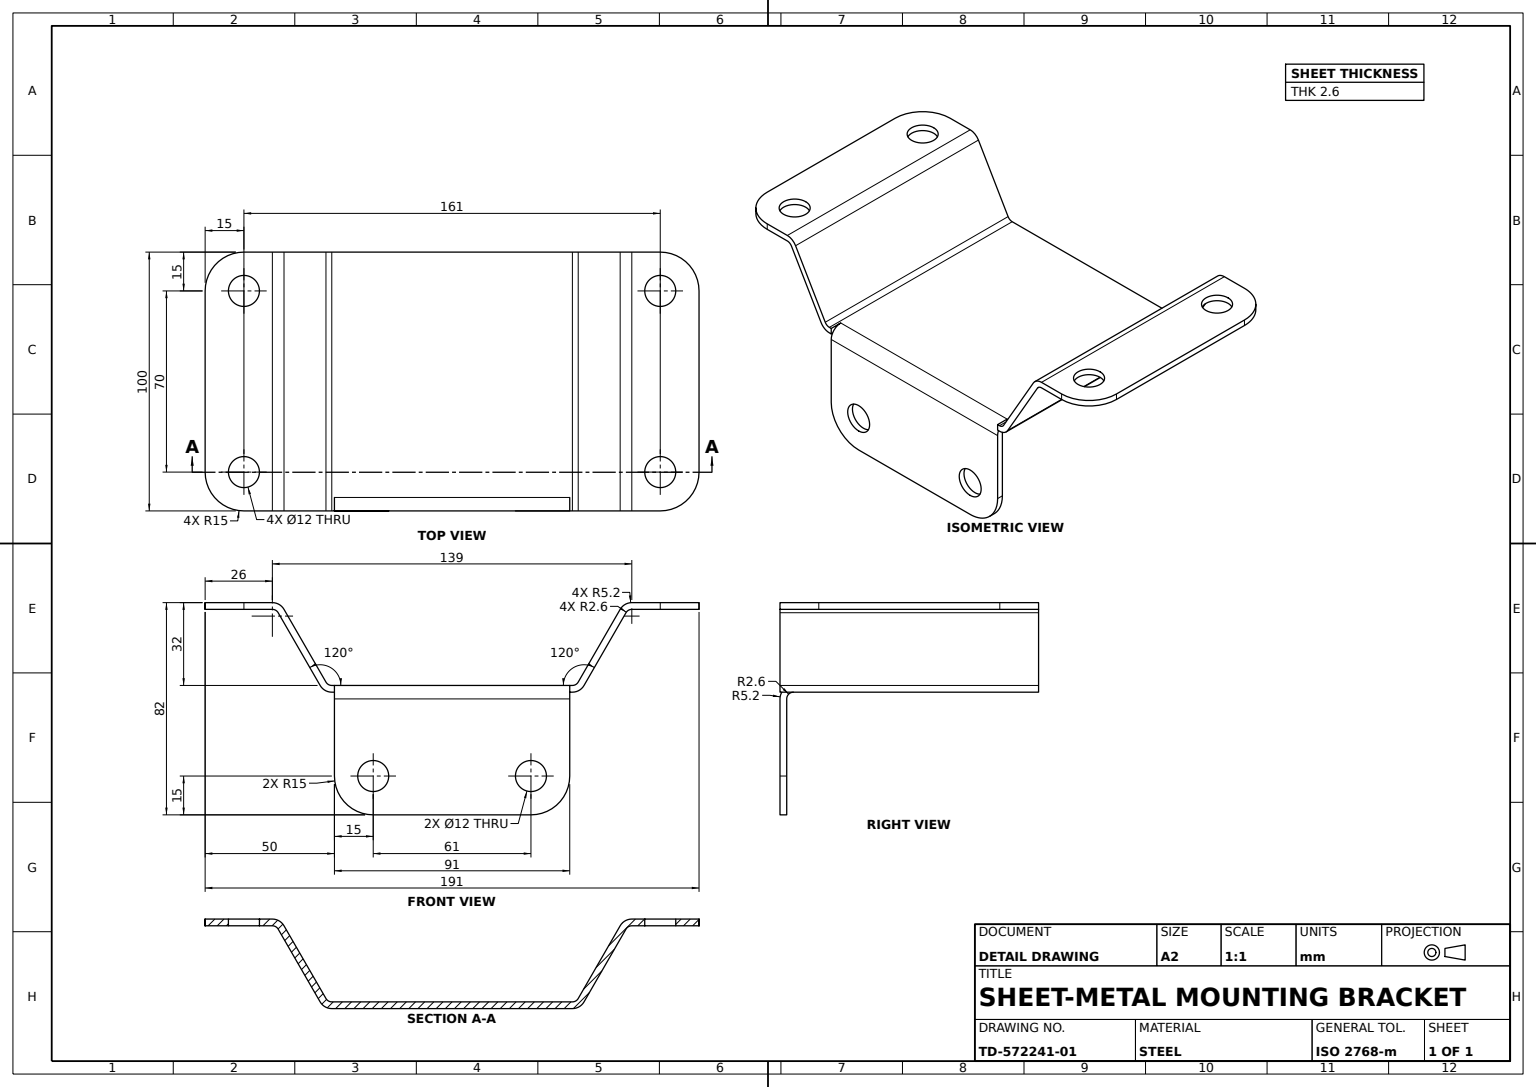
solid
v1 (-51.027013,0,-50)
v2 (-67.250555,28.1,-50)
e1 v1 v2 LINE
v3 (-64.998889,29.4,-50)
e2 v2 v3 LINE
v4 (-48.775347,1.3,-50)
e3 v4 v3 LINE
e4 v4 v1 LINE
face PLANE(AX(P(-46.523681,-2.6,-50),D(0,0,-1),D(-1,0,0))) [e1 e2 -e3 e4]
v5 (-67.250555,28.1,50)
e5 v5 v2 LINE
v6 (-69.502221,29.4,50)
e6 v5 v6 CIRCLE(AX(P(-69.502221,26.8,50),D(0,0,1),D(1,0,0)),2.6)
v7 (-69.502221,29.4,-50)
e7 v6 v7 LINE
e8 v2 v7 CIRCLE(AX(P(-69.502221,26.8,-50),D(0,0,1),D(1,0,0)),2.6)
face CYL(AX(P(-69.502221,26.8,50),D(0,0,-1),D(-1,0,0)),2.6) rev [-e5 e6 e7 -e8]
v8 (45.5,0,50)
v9 (45.5,0,44.8)
e9 v8 v9 LINE
v10 (45.5,-2.6,49.303332)
e10 v9 v10 CIRCLE(AX(P(45.5,-5.2,44.8),D(1,0,0),D(0,0,1)),5.2)
v11 (45.5,-2.6,50)
e11 v10 v11 LINE
e12 v11 v8 LINE
face PLANE(AX(P(45.5,-2.6,44.8),D(-1,0,0),D(0,0,1))) [e9 e10 e11 e12]
v12 (-80.5,29.4,-29)
v13 (-80.5,29.4,-41)
e13 v12 v13 CIRCLE(AX(P(-80.5,29.4,-35),D(0,1,0),D(0,0,1)),6)
v14 (-80.5,32,-29)
e14 v12 v14 LINE
v15 (-80.5,32,-41)
e15 v14 v15 CIRCLE(AX(P(-80.5,32,-35),D(0,1,0),D(0,0,1)),6)
e16 v13 v15 LINE
face CYL(AX(P(-80.5,29.4,-35),D(0,1,0),D(0,0,1)),6) rev [-e13 e14 e15 -e16]
v16 (-64.998889,29.4,50)
v17 (-69.502221,32,50)
e17 v16 v17 CIRCLE(AX(P(-69.502221,26.8,50),D(0,0,1),D(-1,0,0)),5.2)
e18 v16 v3 LINE
v18 (-69.502221,32,-50)
e19 v3 v18 CIRCLE(AX(P(-69.502221,26.8,-50),D(0,0,1),D(-1,0,0)),5.2)
e20 v17 v18 LINE
face CYL(AX(P(-69.502221,26.8,50),D(0,0,-1),D(-1,0,0)),5.2) [-e17 e18 e19 -e20]
v19 (45.5,-5.2,50)
e21 v10 v19 CIRCLE(AX(P(45.5,-5.2,44.8),D(1,0,0),D(0,0,1)),5.2)
v20 (-45.5,0,44.8)
e22 v20 v9 LINE
v21 (-45.5,-2.6,49.303332)
e23 v21 v20 CIRCLE(AX(P(-45.5,-5.2,44.8),D(-1,0,0),D(0,0,1)),5.2)
v22 (-45.5,-5.2,50)
e24 v22 v21 CIRCLE(AX(P(-45.5,-5.2,44.8),D(-1,0,0),D(0,0,1)),5.2)
e25 v22 v19 LINE
face CYL(AX(P(-45.5,-5.2,44.8),D(-1,0,0),D(0,0,1)),5.2) [-e21 -e10 -e22 -e23 -e24 e25]
v23 (51.027013,0,-50)
v24 (48.775347,1.3,-50)
e26 v23 v24 LINE
v25 (46.523681,-2.6,-50)
e27 v23 v25 CIRCLE(AX(P(46.523681,2.6,-50),D(0,0,-1),D(1,0,0)),5.2)
v26 (46.523681,0,-50)
e28 v26 v25 LINE
e29 v24 v26 CIRCLE(AX(P(46.523681,2.6,-50),D(0,0,-1),D(1,0,0)),2.6)
face PLANE(AX(P(46.523681,0,-50),D(0,0,-1),D(-1,0,0))) [-e26 e27 -e28 -e29]
v27 (-95.5,32,35)
v28 (-95.5,32,-35)
e30 v27 v28 LINE
v29 (-95.5,29.4,-35)
e31 v28 v29 LINE
v30 (-95.5,29.4,35)
e32 v30 v29 LINE
e33 v30 v27 LINE
face PLANE(AX(P(-95.5,29.4,50),D(-1,0,0),D(0,0,1))) [e30 e31 -e32 e33]
e34 v16 v5 LINE
v31 (-51.027013,0,50)
e35 v31 v5 LINE
v32 (-48.775347,1.3,50)
e36 v31 v32 LINE
e37 v32 v16 LINE
face PLANE(AX(P(-69.502221,29.4,50),D(0,0,1),D(1,0,0))) [e34 -e35 e36 e37]
v33 (-80.5,32,50)
v34 (-80.5,29.4,50)
e38 v33 v34 LINE
e39 v27 v33 CIRCLE(AX(P(-80.5,32,35),D(0,1,0),D(0,0,-1)),15)
e40 v34 v30 CIRCLE(AX(P(-80.5,29.4,35),D(0,-1,0),D(0,0,-1)),15)
face CYL(AX(P(-80.5,29.4,35),D(0,1,0),D(0,0,1)),15) [-e38 -e39 -e33 -e40]
v35 (-30.5,-41,50)
v36 (-30.5,-29,50)
e41 v35 v36 CIRCLE(AX(P(-30.5,-35,50),D(0,0,-1),D(0,1,0)),6)
v37 (-30.5,-41,47.4)
e42 v35 v37 LINE
v38 (-30.5,-29,47.4)
e43 v37 v38 CIRCLE(AX(P(-30.5,-35,47.4),D(0,0,-1),D(0,1,0)),6)
e44 v36 v38 LINE
face CYL(AX(P(-30.5,-35,50),D(0,0,-1),D(0,1,0)),6) rev [-e41 e42 e43 -e44]
v39 (-80.5,29.4,-50)
e45 v29 v39 CIRCLE(AX(P(-80.5,29.4,-35),D(0,-1,0),D(0,0,-1)),15)
v40 (-80.5,32,-50)
e46 v40 v28 CIRCLE(AX(P(-80.5,32,-35),D(0,1,0),D(0,0,-1)),15)
e47 v39 v40 LINE
face CYL(AX(P(-80.5,28.1,-35),D(0,1,0),D(0,0,1)),15) [-e45 -e31 -e46 -e47]
e48 v36 v35 CIRCLE(AX(P(-30.5,-35,50),D(0,0,-1),D(0,1,0)),6)
v41 (30.5,-29,50)
v42 (30.5,-41,50)
e49 v41 v42 CIRCLE(AX(P(30.5,-35,50),D(0,0,-1),D(0,1,0)),6)
e50 v42 v41 CIRCLE(AX(P(30.5,-35,50),D(0,0,-1),D(0,1,0)),6)
v43 (45.5,-35,50)
v44 (30.5,-50,50)
e51 v43 v44 CIRCLE(AX(P(30.5,-35,50),D(0,0,-1),D(0,1,0)),15)
e52 v19 v43 LINE
v45 (-45.5,-35,50)
e53 v45 v22 LINE
v46 (-30.5,-50,50)
e54 v46 v45 CIRCLE(AX(P(-30.5,-35,50),D(0,0,-1),D(0,1,0)),15)
e55 v44 v46 LINE
face PLANE(AX(P(-30.5,-35,50),D(0,0,-1),D(0,1,0))) rev [e48 e41] [e49 e50] [-e51 -e52 -e25 -e53 -e54 -e55]
v47 (-46.523681,0,50)
v48 (-46.523681,-2.6,50)
e56 v47 v48 LINE
v49 (-45.5,-2.6,50)
e57 v49 v48 LINE
v50 (-45.5,0,50)
e58 v49 v50 LINE
e59 v50 v47 LINE
face PLANE(AX(P(-51.027013,0,50),D(0,0,1),D(1,0,0))) [e56 -e57 e58 e59]
v51 (80.5,29.4,-41)
v52 (80.5,32,-41)
e60 v51 v52 LINE
v53 (80.5,32,-29)
e61 v52 v53 CIRCLE(AX(P(80.5,32,-35),D(0,1,0),D(0,0,1)),6)
v54 (80.5,29.4,-29)
e62 v54 v53 LINE
e63 v51 v54 CIRCLE(AX(P(80.5,29.4,-35),D(0,1,0),D(0,0,1)),6)
face CYL(AX(P(80.5,29.4,-35),D(0,1,0),D(0,0,1)),6) rev [e60 e61 -e62 -e63]
e64 v7 v39 LINE
e65 v18 v40 LINE
e66 v18 v7 LINE
face PLANE(AX(P(-67.250555,28.1,-50),D(0,0,-1),D(-1,0,0))) [e64 e47 -e65 e66]
v55 (46.523681,-2.6,50)
e67 v55 v25 LINE
v56 (51.027013,0,50)
e68 v56 v23 LINE
e69 v56 v55 CIRCLE(AX(P(46.523681,2.6,50),D(0,0,-1),D(1,0,0)),5.2)
face CYL(AX(P(46.523681,2.6,50),D(0,0,-1),D(-1,0,0)),5.2) [e67 -e27 -e68 e69]
e70 v32 v4 LINE
face PLANE(AX(P(-48.024791,0,50),D(-0.866025404,-0.5,0),D(0.5,-0.866025404,0))) rev [e3 -e18 -e37 e70]
v57 (-80.5,29.4,29)
v58 (-80.5,32,29)
e71 v57 v58 LINE
v59 (-80.5,32,41)
e72 v58 v59 CIRCLE(AX(P(-80.5,32,35),D(0,1,0),D(0,0,1)),6)
v60 (-80.5,29.4,41)
e73 v60 v59 LINE
e74 v57 v60 CIRCLE(AX(P(-80.5,29.4,35),D(0,1,0),D(0,0,1)),6)
face CYL(AX(P(-80.5,29.4,35),D(0,1,0),D(0,0,1)),6) rev [e71 e72 -e73 -e74]
v61 (30.5,-50,47.4)
e75 v44 v61 LINE
v62 (45.5,-35,47.4)
e76 v62 v61 CIRCLE(AX(P(30.5,-35,47.4),D(0,0,-1),D(0,1,0)),15)
e77 v43 v62 LINE
face CYL(AX(P(30.5,-35,50),D(0,0,-1),D(0,1,0)),15) [e75 -e76 -e77 e51]
v63 (64.998889,29.4,-50)
v64 (67.250555,28.1,-50)
e78 v63 v64 LINE
v65 (69.502221,32,-50)
e79 v65 v63 CIRCLE(AX(P(69.502221,26.8,-50),D(0,0,1),D(-1,0,0)),5.2)
v66 (69.502221,29.4,-50)
e80 v66 v65 LINE
e81 v66 v64 CIRCLE(AX(P(69.502221,26.8,-50),D(0,0,1),D(1,0,0)),2.6)
face PLANE(AX(P(64.998889,29.4,-50),D(0,0,-1),D(-1,0,0))) [-e78 -e79 -e80 e81]
e82 v21 v49 LINE
e83 v50 v20 LINE
face PLANE(AX(P(-45.5,-2.6,44.8),D(-1,0,0),D(0,0,1))) rev [-e82 e23 -e83 -e58]
e84 v31 v1 LINE
face PLANE(AX(P(-50.276457,-1.3,50),D(-0.866025404,-0.5,0),D(0.5,-0.866025404,0))) [e5 -e1 -e84 e35]
v67 (30.5,-41,47.4)
v68 (30.5,-29,47.4)
e85 v67 v68 CIRCLE(AX(P(30.5,-35,47.4),D(0,0,-1),D(0,1,0)),6)
e86 v41 v68 LINE
e87 v42 v67 LINE
face CYL(AX(P(30.5,-35,50),D(0,0,-1),D(0,1,0)),6) rev [e85 -e86 -e50 e87]
v69 (80.5,32,41)
v70 (80.5,32,29)
e88 v69 v70 CIRCLE(AX(P(80.5,32,35),D(0,1,0),D(0,0,1)),6)
v71 (80.5,29.4,29)
e89 v71 v70 LINE
v72 (80.5,29.4,41)
e90 v72 v71 CIRCLE(AX(P(80.5,29.4,35),D(0,1,0),D(0,0,1)),6)
e91 v72 v69 LINE
face CYL(AX(P(80.5,29.4,35),D(0,1,0),D(0,0,1)),6) rev [e88 -e89 -e90 e91]
v73 (46.523681,0,50)
e92 v73 v8 LINE
e93 v55 v11 LINE
e94 v55 v73 LINE
face PLANE(AX(P(-51.027013,0,50),D(0,0,1),D(1,0,0))) [e92 -e12 -e93 e94]
e95 v13 v12 CIRCLE(AX(P(-80.5,29.4,-35),D(0,1,0),D(0,0,1)),6)
e96 v15 v14 CIRCLE(AX(P(-80.5,32,-35),D(0,1,0),D(0,0,1)),6)
face CYL(AX(P(-80.5,29.4,-35),D(0,1,0),D(0,0,1)),6) rev [-e95 e16 e96 -e14]
v74 (69.502221,32,50)
e97 v74 v65 LINE
v75 (64.998889,29.4,50)
e98 v75 v63 LINE
e99 v74 v75 CIRCLE(AX(P(69.502221,26.8,50),D(0,0,1),D(-1,0,0)),5.2)
face CYL(AX(P(69.502221,26.8,50),D(0,0,-1),D(-1,0,0)),5.2) [e97 e79 -e98 -e99]
v76 (-46.523681,0,-50)
e100 v26 v76 LINE
e101 v47 v76 LINE
e102 v73 v26 LINE
face PLANE(AX(P(-48.024791,0,50),D(0,-1,0),D(0,0,-1))) rev [e100 -e101 -e59 e83 e22 -e9 -e92 e102]
face PLANE(AX(P(-69.502221,32,-50),D(0,0,-1),D(-1,0,0))) [e8 -e66 -e19 -e2]
v77 (-30.5,-50,47.4)
e103 v46 v77 LINE
e104 v61 v77 LINE
face PLANE(AX(P(-30.5,-50,50),D(0,-1,0),D(0,0,-1))) [e103 -e104 -e75 e55]
e105 v17 v33 LINE
e106 v59 v58 CIRCLE(AX(P(-80.5,32,35),D(0,1,0),D(0,0,1)),6)
face PLANE(AX(P(-66.5,32,50),D(0,-1,0),D(0,0,-1))) rev [-e105 e20 e65 e46 -e30 e39] [-e96 -e15] [-e106 -e72]
e107 v68 v67 CIRCLE(AX(P(30.5,-35,47.4),D(0,0,-1),D(0,1,0)),6)
e108 v38 v37 CIRCLE(AX(P(-30.5,-35,47.4),D(0,0,-1),D(0,1,0)),6)
v78 (-45.5,-35,47.4)
e109 v77 v78 CIRCLE(AX(P(-30.5,-35,47.4),D(0,0,-1),D(0,1,0)),15)
v79 (-45.5,-5.2,47.4)
e110 v78 v79 LINE
v80 (45.5,-5.2,47.4)
e111 v80 v79 LINE
e112 v80 v62 LINE
face PLANE(AX(P(-30.5,-35,47.4),D(0,0,-1),D(0,1,0))) [-e107 -e85] [-e43 -e108] [e104 e109 e110 -e111 e112 e76]
v81 (80.5,32,50)
e113 v81 v74 LINE
v82 (69.502221,29.4,50)
e114 v74 v82 LINE
v83 (80.5,29.4,50)
e115 v83 v82 LINE
e116 v83 v81 LINE
face PLANE(AX(P(67.250555,28.1,50),D(0,0,1),D(1,0,0))) [e113 e114 -e115 e116]
e117 v64 v23 LINE
e118 v63 v24 LINE
face PLANE(AX(P(69.502221,29.4,-50),D(0,0,-1),D(-1,0,0))) [e117 e26 -e118 e78]
v84 (67.250555,28.1,50)
e119 v84 v75 LINE
e120 v82 v84 CIRCLE(AX(P(69.502221,26.8,50),D(0,0,1),D(1,0,0)),2.6)
face PLANE(AX(P(69.502221,32,50),D(0,0,1),D(1,0,0))) [-e119 -e120 -e114 e99]
e121 v71 v72 CIRCLE(AX(P(80.5,29.4,35),D(0,1,0),D(0,0,1)),6)
e122 v70 v69 CIRCLE(AX(P(80.5,32,35),D(0,1,0),D(0,0,1)),6)
face CYL(AX(P(80.5,29.4,35),D(0,1,0),D(0,0,1)),6) rev [-e91 -e121 e89 e122]
e123 v80 v19 LINE
v85 (45.5,-2.6,44.8)
e124 v85 v80 CIRCLE(AX(P(45.5,-5.2,44.8),D(1,0,0),D(0,0,1)),2.6)
e125 v85 v10 LINE
face PLANE(AX(P(45.5,-5.2,44.8),D(1,0,0),D(0,0,-1))) [-e123 -e124 e125 e21]
e126 v6 v34 LINE
e127 v6 v17 LINE
face PLANE(AX(P(-69.502221,26.8,50),D(0,0,1),D(1,0,0))) [e38 -e126 e127 e105]
v86 (48.775347,1.3,50)
e128 v86 v73 CIRCLE(AX(P(46.523681,2.6,50),D(0,0,-1),D(1,0,0)),2.6)
e129 v86 v24 LINE
face CYL(AX(P(46.523681,2.6,50),D(0,0,-1),D(-1,0,0)),2.6) rev [-e128 e129 e29 -e102]
e130 v86 v56 LINE
face PLANE(AX(P(48.775347,1.3,50),D(0,0,1),D(1,0,0))) [e128 -e94 -e69 -e130]
v87 (95.5,32,-35)
v88 (80.5,32,-50)
e131 v87 v88 CIRCLE(AX(P(80.5,32,-35),D(0,1,0),D(0,0,-1)),15)
e132 v88 v65 LINE
v89 (95.5,32,35)
e133 v81 v89 CIRCLE(AX(P(80.5,32,35),D(0,1,0),D(0,0,-1)),15)
e134 v89 v87 LINE
e135 v53 v52 CIRCLE(AX(P(80.5,32,-35),D(0,1,0),D(0,0,1)),6)
face PLANE(AX(P(66.5,32,50),D(0,-1,0),D(0,0,-1))) rev [e131 e132 -e97 -e113 e133 e134] [-e61 -e135] [-e88 -e122]
face CYL(AX(P(-30.5,-35,50),D(0,0,-1),D(0,1,0)),6) rev [-e48 e44 e108 -e42]
v90 (-45.5,-2.6,44.8)
e136 v90 v85 LINE
e137 v90 v21 LINE
v91 (-46.523681,-2.6,-50)
e138 v48 v91 LINE
e139 v25 v91 LINE
face PLANE(AX(P(-48.024791,-2.6,50),D(0,-1,0),D(0,0,-1))) [-e136 e137 e82 e57 e138 -e139 -e67 e93 -e11 -e125]
v92 (95.5,29.4,35)
e140 v89 v92 LINE
e141 v92 v83 CIRCLE(AX(P(80.5,29.4,35),D(0,-1,0),D(0,0,-1)),15)
face CYL(AX(P(80.5,32,35),D(0,-1,0),D(0,0,-1)),15) [-e140 -e133 -e116 -e141]
face PLANE(AX(P(-64.998889,29.4,50),D(0,0,1),D(1,0,0))) [-e127 -e6 -e34 e17]
e142 v84 v56 LINE
e143 v84 v64 LINE
face PLANE(AX(P(50.276457,-1.3,50),D(0.866025404,-0.5,0),D(0.5,0.866025404,0))) [e142 e68 -e117 -e143]
e144 v47 v32 CIRCLE(AX(P(-46.523681,2.6,50),D(0,0,-1),D(1,0,0)),2.6)
e145 v48 v31 CIRCLE(AX(P(-46.523681,2.6,50),D(0,0,-1),D(1,0,0)),5.2)
face PLANE(AX(P(-46.523681,0,50),D(0,0,1),D(1,0,0))) [e144 -e36 -e145 -e56]
e146 v45 v78 LINE
face CYL(AX(P(-30.5,-35,50),D(0,0,-1),D(0,1,0)),15) [e146 -e109 -e103 e54]
e147 v75 v86 LINE
face PLANE(AX(P(46.523681,-2.6,50),D(0,0,1),D(1,0,0))) [e147 e130 -e142 e119]
e148 v79 v90 CIRCLE(AX(P(-45.5,-5.2,44.8),D(-1,0,0),D(0,0,1)),2.6)
face CYL(AX(P(-45.5,-5.2,44.8),D(-1,0,0),D(0,0,1)),2.6) rev [e111 e148 e136 e124]
e149 v54 v51 CIRCLE(AX(P(80.5,29.4,-35),D(0,1,0),D(0,0,1)),6)
face CYL(AX(P(80.5,29.4,-35),D(0,1,0),D(0,0,1)),6) rev [-e149 e62 e135 -e60]
face CYL(AX(P(30.5,-35,50),D(0,0,-1),D(0,1,0)),6) rev [e107 -e87 -e49 e86]
e150 v82 v66 LINE
face CYL(AX(P(69.502221,26.8,50),D(0,0,-1),D(-1,0,0)),2.6) rev [e143 -e81 -e150 e120]
e151 v76 v4 CIRCLE(AX(P(-46.523681,2.6,-50),D(0,0,-1),D(1,0,0)),2.6)
e152 v91 v76 LINE
e153 v91 v1 CIRCLE(AX(P(-46.523681,2.6,-50),D(0,0,-1),D(1,0,0)),5.2)
face PLANE(AX(P(-48.775347,1.3,-50),D(0,0,-1),D(-1,0,0))) [-e4 -e151 -e152 e153]
face PLANE(AX(P(51.027013,0,-50),D(0,0,-1),D(-1,0,0))) [e139 e152 -e100 e28]
face CYL(AX(P(-46.523681,2.6,50),D(0,0,-1),D(-1,0,0)),5.2) [-e138 e145 e84 -e153]
v93 (80.5,29.4,-50)
e154 v88 v93 LINE
e155 v93 v66 LINE
face PLANE(AX(P(-69.502221,26.8,-50),D(0,0,1),D(1,0,0))) rev [e80 -e132 e154 e155]
e156 v79 v22 LINE
face PLANE(AX(P(-45.5,-5.2,44.8),D(1,0,0),D(0,0,-1))) rev [e156 e24 -e137 -e148]
face PLANE(AX(P(-45.5,-2.6,50),D(-1,0,0),D(0,-1,0))) [e53 -e156 -e110 -e146]
v94 (95.5,29.4,-35)
e157 v94 v87 LINE
e158 v92 v94 LINE
face PLANE(AX(P(95.5,32,50),D(1,0,0),D(0,0,-1))) [e157 -e134 e140 e158]
face CYL(AX(P(-46.523681,2.6,50),D(0,0,-1),D(-1,0,0)),2.6) rev [-e144 e101 e151 -e70]
e159 v93 v94 CIRCLE(AX(P(80.5,29.4,-35),D(0,-1,0),D(0,0,-1)),15)
face PLANE(AX(P(66.5,29.4,50),D(0,-1,0),D(0,0,-1))) [e63 e149] [e115 e150 -e155 e159 -e158 e141] [e90 e121]
e160 v60 v57 CIRCLE(AX(P(-80.5,29.4,35),D(0,1,0),D(0,0,1)),6)
face PLANE(AX(P(-66.5,29.4,50),D(0,-1,0),D(0,0,-1))) [e126 e40 e32 e45 -e64 -e7] [e160 e74] [e13 e95]
face CYL(AX(P(80.5,26.8,-35),D(0,1,0),D(0,0,1)),15) [-e159 -e154 -e131 -e157]
face PLANE(AX(P(48.024791,0,50),D(0.866025404,-0.5,0),D(0.5,0.866025404,0))) rev [-e129 -e147 e98 e118]
face PLANE(AX(P(45.5,-35,50),D(1,0,0),D(0,1,0))) [e123 e52 e77 -e112]
face CYL(AX(P(-80.5,29.4,35),D(0,1,0),D(0,0,1)),6) rev [e73 e106 -e71 -e160]
